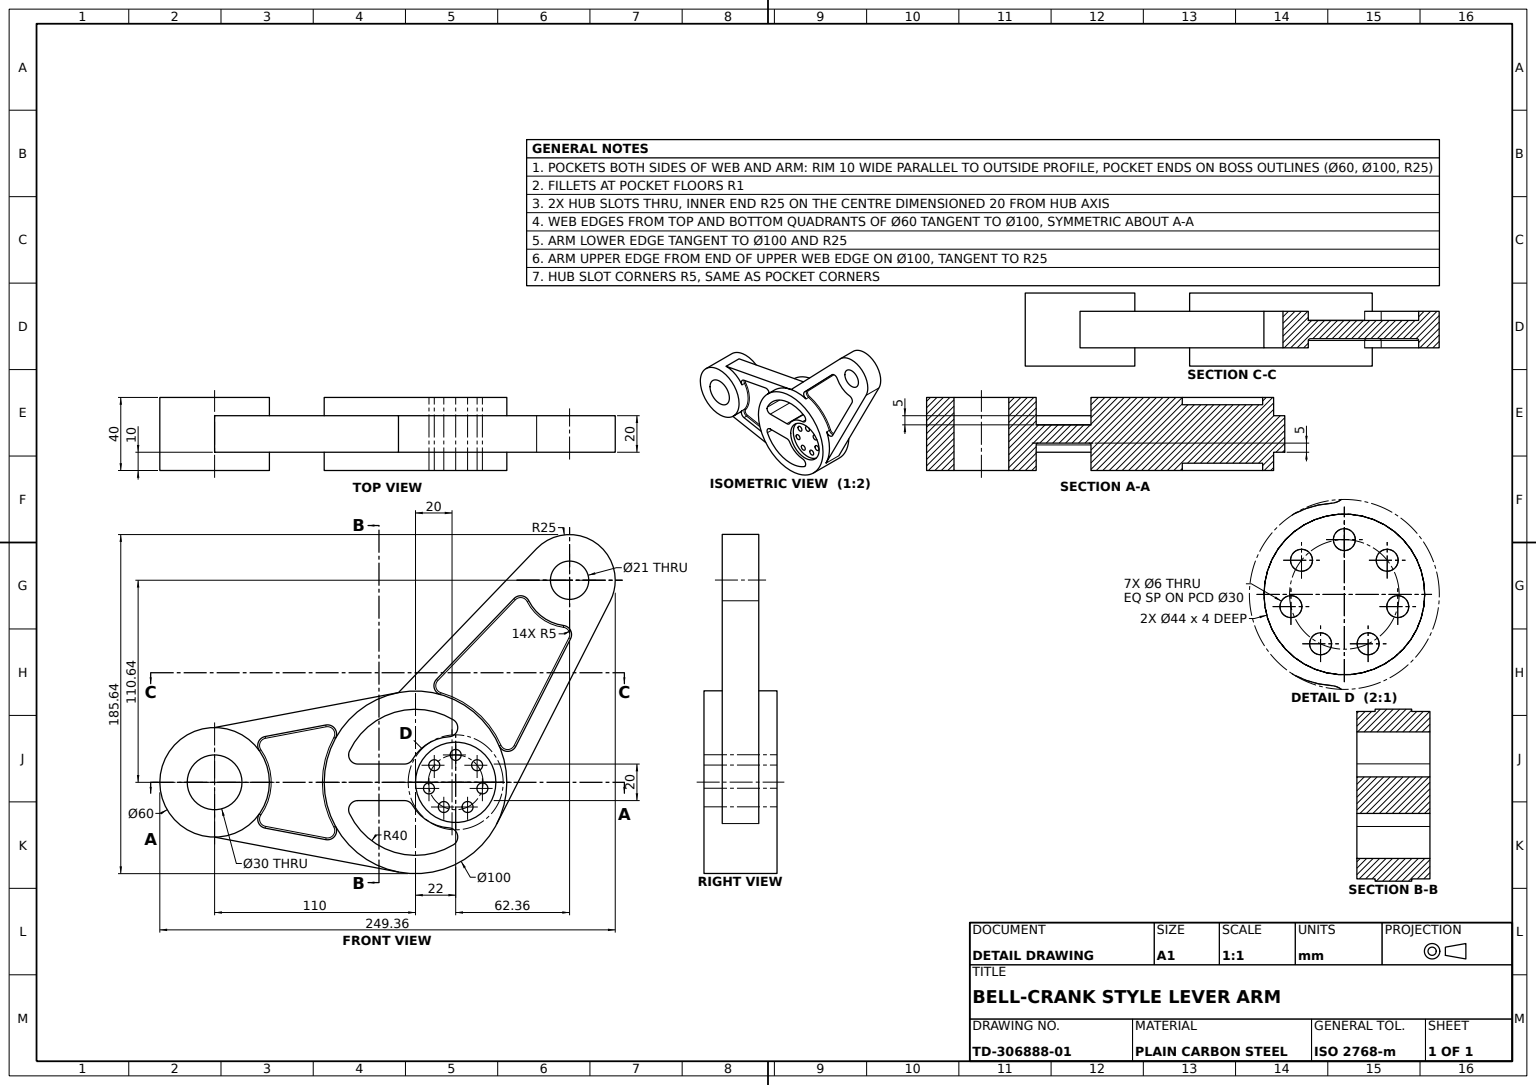
solid
v1 (18.491743913,-13.514533019,4)
v2 (18.491743913,-13.514533019,36)
e1 v1 v2 LINE
v3 (12.491743913,-13.514533019,36)
e2 v2 v3 CIRCLE(AX(P(15.491743913,-13.514533019,36),D(0,0,1),D(1,0,0)),3)
v4 (12.491743913,-13.514533019,4)
e3 v4 v3 LINE
e4 v4 v1 CIRCLE(AX(P(15.491743913,-13.514533019,4),D(0,0,-1),D(-1,0,0)),3)
face CYL(AX(P(15.491743913,-13.514533019,-4),D(0,0,1),D(1,0,0)),3) rev [e1 e2 -e3 e4]
v5 (54.673235414,99.92377456,25)
v6 (12.193310999,55.662253979,25)
e5 v5 v6 LINE
v7 (53.95175742,100.616211925,26)
e6 v7 v5 CIRCLE(AX(P(54.673235414,99.92377456,26),D(-0.692437365,-0.721477994,0),D(0.721477994,-0.692437365,0)),1)
v8 (11.471833004,56.354691343,26)
e7 v8 v7 LINE
e8 v8 v6 CIRCLE(AX(P(12.193310999,55.662253979,26),D(-0.692437365,-0.721477994,0),D(0.721477994,-0.692437365,0)),1)
face CYL(AX(P(12.193310999,55.662253979,26),D(-0.692437365,-0.721477994,0),D(0.721477994,-0.692437365,0)),1) rev [-e5 -e6 -e7 e8]
v9 (-36.622776602,15,40)
v10 (-36.622776602,15,0)
e9 v9 v10 LINE
v11 (-31.622776602,10,40)
e10 v11 v9 CIRCLE(AX(P(-31.622776602,15,40),D(0,0,-1),D(1,0,0)),5)
v12 (-31.622776602,10,0)
e11 v11 v12 LINE
e12 v12 v10 CIRCLE(AX(P(-31.622776602,15,0),D(0,0,-1),D(1,0,0)),5)
face CYL(AX(P(-31.622776602,15,40),D(0,0,-1),D(-1,0,0)),5) rev [-e9 -e10 e11 e12]
v13 (10.376081317,-3.337814009,36)
v14 (4.376081317,-3.337814009,36)
e13 v13 v14 CIRCLE(AX(P(7.376081317,-3.337814009,36),D(0,0,1),D(1,0,0)),3)
e14 v14 v13 CIRCLE(AX(P(7.376081317,-3.337814009,36),D(0,0,1),D(1,0,0)),3)
e15 v3 v2 CIRCLE(AX(P(15.491743913,-13.514533019,36),D(0,0,1),D(1,0,0)),3)
v15 (13.272527763,9.352347028,36)
v16 (7.272527763,9.352347028,36)
e16 v15 v16 CIRCLE(AX(P(10.272527763,9.352347028,36),D(0,0,1),D(1,0,0)),3)
e17 v16 v15 CIRCLE(AX(P(10.272527763,9.352347028,36),D(0,0,1),D(1,0,0)),3)
v17 (39.623918683,-3.337814009,36)
v18 (33.623918683,-3.337814009,36)
e18 v17 v18 CIRCLE(AX(P(36.623918683,-3.337814009,36),D(0,0,1),D(1,0,0)),3)
e19 v18 v17 CIRCLE(AX(P(36.623918683,-3.337814009,36),D(0,0,1),D(1,0,0)),3)
v19 (31.508256087,-13.514533019,36)
v20 (25.508256087,-13.514533019,36)
e20 v19 v20 CIRCLE(AX(P(28.508256087,-13.514533019,36),D(0,0,1),D(1,0,0)),3)
e21 v20 v19 CIRCLE(AX(P(28.508256087,-13.514533019,36),D(0,0,1),D(1,0,0)),3)
v21 (25,15,36)
v22 (19,15,36)
e22 v21 v22 CIRCLE(AX(P(22,15,36),D(0,0,1),D(1,0,0)),3)
e23 v22 v21 CIRCLE(AX(P(22,15,36),D(0,0,1),D(1,0,0)),3)
v23 (0,0,36)
v24 (44,0,36)
e24 v23 v24 CIRCLE(AX(P(22,0,36),D(0,0,1),D(1,0,0)),22)
e25 v24 v23 CIRCLE(AX(P(22,0,36),D(0,0,1),D(1,0,0)),22)
v25 (36.727472237,9.352347028,36)
v26 (30.727472237,9.352347028,36)
e26 v25 v26 CIRCLE(AX(P(33.727472237,9.352347028,36),D(0,0,1),D(1,0,0)),3)
e27 v26 v25 CIRCLE(AX(P(33.727472237,9.352347028,36),D(0,0,1),D(1,0,0)),3)
face PLANE(AX(P(22,0,36),D(0,0,1),D(1,0,0))) [-e13 -e14] [-e2 -e15] [-e16 -e17] [-e18 -e19] [-e20 -e21] [-e22 -e23] [e24 e25] [-e26 -e27]
v27 (81.094875761,85.850138645,30)
v28 (84.898130502,78.625049023,30)
e28 v27 v28 CIRCLE(AX(P(80.442048198,80.892940225,30),D(0,0,-1),D(1,0,0)),5)
v29 (81.094875761,85.850138645,26)
e29 v27 v29 LINE
v30 (85.442048198,80.892940225,26)
e30 v29 v30 CIRCLE(AX(P(80.442048198,80.892940225,26),D(0,0,-1),D(1,0,0)),5)
v31 (84.898130502,78.625049023,26)
e31 v30 v31 CIRCLE(AX(P(80.442048198,80.892940225,26),D(0,0,-1),D(1,0,0)),5)
e32 v28 v31 LINE
face CYL(AX(P(80.442048198,80.892940225,30),D(0,0,-1),D(-1,0,0)),5) rev [-e28 e29 e30 e31 -e32]
v32 (53.95175742,100.616211925,30)
e33 v32 v7 LINE
v33 (62.025791755,99.401042709,26)
e34 v7 v33 CIRCLE(AX(P(57.559147391,97.154025102,26),D(0,0,-1),D(1,0,0)),5)
v34 (62.025791755,99.401042709,30)
e35 v34 v33 LINE
e36 v32 v34 CIRCLE(AX(P(57.559147391,97.154025102,30),D(0,0,-1),D(1,0,0)),5)
face CYL(AX(P(57.559147391,97.154025102,30),D(0,0,-1),D(-1,0,0)),5) rev [e33 e34 -e35 -e36]
v35 (-82.326208539,25.077710319,30)
v36 (-82.326208539,25.077710319,26)
e37 v35 v36 LINE
v37 (-49.145510288,31.38022974,26)
e38 v36 v37 LINE
v38 (-49.145510288,31.38022974,30)
e39 v38 v37 LINE
e40 v35 v38 LINE
face PLANE(AX(P(-7.464353139,39.297371823,30),D(-0.186608828,0.982434296,0),D(-0.982434296,-0.186608828,0))) rev [e37 e38 -e39 -e40]
v39 (44,0,4)
v40 (44,0,0)
e41 v39 v40 LINE
v41 (0,0,4)
e42 v41 v39 CIRCLE(AX(P(22,0,4),D(0,0,-1),D(-1,0,0)),22)
v42 (0,0,0)
e43 v41 v42 LINE
e44 v42 v40 CIRCLE(AX(P(22,0,0),D(0,0,-1),D(-1,0,0)),22)
face CYL(AX(P(22,0,4),D(0,0,-1),D(-1,0,0)),22) rev [-e41 -e42 e43 e44]
v43 (-82.326208539,-25.077710319,26)
v44 (-86.393164396,-20.165538841,26)
e45 v43 v44 CIRCLE(AX(P(-81.393164396,-20.165538841,26),D(0,0,-1),D(-1,0,0)),5)
v45 (-86.393164396,-20.165538841,30)
e46 v45 v44 LINE
v46 (-82.326208539,-25.077710319,30)
e47 v46 v45 CIRCLE(AX(P(-81.393164396,-20.165538841,30),D(0,0,-1),D(1,0,0)),5)
e48 v46 v43 LINE
face CYL(AX(P(-81.393164396,-20.165538841,30),D(0,0,-1),D(-1,0,0)),5) rev [e45 -e46 -e47 e48]
v47 (-49.145510288,-31.38022974,30)
e49 v46 v47 LINE
v48 (-85.479855197,-17.284747578,30)
e50 v45 v48 CIRCLE(AX(P(-81.393164396,-20.165538841,30),D(0,0,-1),D(1,0,0)),5)
v49 (-110,-30,30)
e51 v48 v49 CIRCLE(AX(P(-110,0,30),D(0,0,-1),D(1,0,0)),30)
v50 (-9.330441424,-49.121714779,30)
e52 v49 v50 LINE
v51 (-43.829514678,-24.061871148,30)
e53 v51 v50 CIRCLE(AX(P(0,0,30),D(0,0,1),D(1,0,0)),50)
e54 v47 v51 CIRCLE(AX(P(-48.212466145,-26.468058263,30),D(0,0,1),D(1,0,0)),5)
face PLANE(AX(P(0,0,30),D(0,0,1),D(1,0,0))) [-e49 e47 e50 e51 e52 -e53 -e54]
v52 (-86.393164396,20.165538841,26)
e55 v52 v36 CIRCLE(AX(P(-81.393164396,20.165538841,26),D(0,0,-1),D(-1,0,0)),5)
v53 (-86.393164396,20.165538841,30)
e56 v35 v53 CIRCLE(AX(P(-81.393164396,20.165538841,30),D(0,0,1),D(1,0,0)),5)
e57 v53 v52 LINE
face CYL(AX(P(-81.393164396,20.165538841,30),D(0,0,-1),D(-1,0,0)),5) rev [e55 -e37 e56 e57]
v54 (33.623918683,-3.337814009,4)
e58 v54 v18 LINE
v55 (39.623918683,-3.337814009,4)
e59 v54 v55 CIRCLE(AX(P(36.623918683,-3.337814009,4),D(0,0,-1),D(-1,0,0)),3)
e60 v55 v17 LINE
face CYL(AX(P(36.623918683,-3.337814009,-4),D(0,0,1),D(1,0,0)),3) rev [e18 -e58 e59 e60]
v56 (-85.479855197,-17.284747578,15)
v57 (-85.479855197,-17.284747578,10)
e61 v56 v57 LINE
v58 (-86.393164396,-20.165538841,15)
e62 v56 v58 CIRCLE(AX(P(-81.393164396,-20.165538841,15),D(0,0,1),D(1,0,0)),5)
v59 (-86.393164396,-20.165538841,10)
e63 v58 v59 LINE
e64 v59 v57 CIRCLE(AX(P(-81.393164396,-20.165538841,10),D(0,0,-1),D(1,0,0)),5)
face CYL(AX(P(-81.393164396,-20.165538841,30),D(0,0,-1),D(-1,0,0)),5) rev [-e61 e62 e63 e64]
v60 (11.471833004,56.354691343,30)
v61 (10.079222976,52.892504521,30)
e65 v60 v61 CIRCLE(AX(P(15.079222976,52.892504521,30),D(0,0,1),D(1,0,0)),5)
v62 (10.079222976,52.892504521,26)
e66 v61 v62 LINE
e67 v62 v8 CIRCLE(AX(P(15.079222976,52.892504521,26),D(0,0,-1),D(1,0,0)),5)
e68 v60 v8 LINE
face CYL(AX(P(15.079222976,52.892504521,30),D(0,0,-1),D(-1,0,0)),5) rev [e65 e66 e67 -e68]
v63 (11.471833004,56.354691343,15)
v64 (11.471833004,56.354691343,10)
e69 v63 v64 LINE
v65 (10.079222976,52.892504521,15)
e70 v63 v65 CIRCLE(AX(P(15.079222976,52.892504521,15),D(0,0,1),D(1,0,0)),5)
v66 (10.079222976,52.892504521,10)
e71 v65 v66 LINE
e72 v64 v66 CIRCLE(AX(P(15.079222976,52.892504521,10),D(0,0,1),D(1,0,0)),5)
face CYL(AX(P(15.079222976,52.892504521,30),D(0,0,-1),D(-1,0,0)),5) rev [-e69 e70 e71 -e72]
v67 (-85.393164396,-20.165538841,25)
v68 (-82.13959971,-24.095276023,25)
e73 v67 v68 CIRCLE(AX(P(-81.393164396,-20.165538841,25),D(0,0,1),D(-1,0,0)),4)
e74 v44 v67 CIRCLE(AX(P(-85.393164396,-20.165538841,26),D(0,-1,0),D(0,0,-1)),1)
e75 v68 v43 CIRCLE(AX(P(-82.13959971,-24.095276023,26),D(-0.982434296,0.186608828,0),D(-0.186608828,-0.982434296,0)),1)
face TORUS(AX(P(-81.393164396,-20.165538841,26),D(0,0,-1),D(-1,0,0)),4,1) rev [-e73 -e74 -e45 -e75]
v69 (-36.140316116,-17.142857143,40)
v70 (-36.140316116,-17.142857143,0)
e76 v69 v70 LINE
v71 (-36.622776602,-15,0)
e77 v71 v70 CIRCLE(AX(P(-31.622776602,-15,0),D(0,0,1),D(1,0,0)),5)
v72 (-36.622776602,-15,40)
e78 v72 v71 LINE
e79 v72 v69 CIRCLE(AX(P(-31.622776602,-15,40),D(0,0,1),D(1,0,0)),5)
face CYL(AX(P(-31.622776602,-15,40),D(0,0,-1),D(-1,0,0)),5) rev [e76 -e77 -e78 e79]
v73 (-36.140316116,17.142857143,40)
v74 (-36.140316116,17.142857143,0)
e80 v73 v74 LINE
v75 (20.714285714,34.218684477,0)
e81 v75 v74 CIRCLE(AX(P(0,0,0),D(0,0,1),D(1,0,0)),40)
v76 (20.714285714,34.218684477,40)
e82 v76 v75 LINE
e83 v76 v73 CIRCLE(AX(P(0,0,40),D(0,0,1),D(1,0,0)),40)
face CYL(AX(P(0,0,40),D(0,0,-1),D(-1,0,0)),40) rev [e80 -e81 -e82 e83]
v77 (13.272527763,9.352347028,4)
e84 v77 v15 LINE
v78 (7.272527763,9.352347028,4)
e85 v77 v78 CIRCLE(AX(P(10.272527763,9.352347028,4),D(0,0,-1),D(-1,0,0)),3)
e86 v78 v16 LINE
face CYL(AX(P(10.272527763,9.352347028,-4),D(0,0,1),D(1,0,0)),3) rev [e17 -e84 e85 e86]
v79 (-85.479855197,17.284747578,30)
e87 v53 v79 CIRCLE(AX(P(-81.393164396,20.165538841,30),D(0,0,1),D(1,0,0)),5)
v80 (-85.479855197,17.284747578,26)
e88 v79 v80 LINE
e89 v80 v52 CIRCLE(AX(P(-81.393164396,20.165538841,26),D(0,0,-1),D(-1,0,0)),5)
face CYL(AX(P(-81.393164396,20.165538841,30),D(0,0,-1),D(-1,0,0)),5) rev [e87 e88 e89 -e57]
v81 (-82.326208539,-25.077710319,15)
v82 (-49.145510288,-31.38022974,15)
e90 v81 v82 LINE
v83 (-49.145510288,-31.38022974,10)
e91 v82 v83 LINE
v84 (-82.326208539,-25.077710319,10)
e92 v84 v83 LINE
e93 v81 v84 LINE
face PLANE(AX(P(-7.464353139,-39.297371823,30),D(0.186608828,0.982434296,0),D(-0.982434296,0.186608828,0))) [e90 e91 -e92 -e93]
v85 (13.708384523,48.084095019,30)
e94 v61 v85 CIRCLE(AX(P(15.079222976,52.892504521,30),D(0,0,1),D(1,0,0)),5)
v86 (13.708384523,48.084095019,26)
e95 v85 v86 LINE
e96 v86 v62 CIRCLE(AX(P(15.079222976,52.892504521,26),D(0,0,-1),D(1,0,0)),5)
face CYL(AX(P(15.079222976,52.892504521,30),D(0,0,-1),D(-1,0,0)),5) rev [-e66 e94 e95 e96]
e97 v78 v77 CIRCLE(AX(P(10.272527763,9.352347028,4),D(0,0,-1),D(-1,0,0)),3)
face CYL(AX(P(10.272527763,9.352347028,-4),D(0,0,1),D(1,0,0)),3) rev [-e86 e97 e84 e16]
v87 (-5.980762114,-10,40)
v88 (-5.980762114,-10,0)
e98 v87 v88 LINE
v89 (-31.622776602,-10,40)
e99 v87 v89 LINE
v90 (-31.622776602,-10,0)
e100 v89 v90 LINE
e101 v88 v90 LINE
face PLANE(AX(P(0,-10,40),D(0,-1,0),D(1,0,0))) [-e98 e99 e100 -e101]
v91 (13.708384523,48.084095019,15)
v92 (13.708384523,48.084095019,10)
e102 v91 v92 LINE
e103 v66 v92 CIRCLE(AX(P(15.079222976,52.892504521,10),D(0,0,1),D(1,0,0)),5)
e104 v65 v91 CIRCLE(AX(P(15.079222976,52.892504521,15),D(0,0,1),D(1,0,0)),5)
face CYL(AX(P(15.079222976,52.892504521,30),D(0,0,-1),D(-1,0,0)),5) rev [e102 -e103 -e71 e104]
v93 (45.851155545,19.941703417,26)
v94 (46.768178656,20.340537485,25)
e105 v93 v94 CIRCLE(AX(P(46.768178656,20.340537485,26),D(0.398834068,-0.917023111,0),D(0.917023111,0.398834068,0)),1)
v95 (54.892353403,19.667982557,26)
e106 v95 v93 CIRCLE(AX(P(50.4362711,21.935873759,26),D(0,0,-1),D(1,0,0)),5)
v96 (54.001136943,20.121560797,25)
e107 v96 v95 CIRCLE(AX(P(54.001136943,20.121560797,26),D(-0.45357824,-0.891216461,0),D(0.891216461,-0.45357824,0)),1)
e108 v94 v96 CIRCLE(AX(P(50.4362711,21.935873759,25),D(0,0,1),D(1,0,0)),4)
face TORUS(AX(P(50.4362711,21.935873759,26),D(0,0,1),D(1,0,0)),4,1) rev [-e105 -e106 -e107 -e108]
v97 (-50,0,26)
v98 (-43.829514678,-24.061871148,26)
e109 v97 v98 CIRCLE(AX(P(0,0,26),D(0,0,1),D(-1,0,0)),50)
v99 (-51,0,25)
e110 v99 v97 CIRCLE(AX(P(-51,0,26),D(0,-1,0),D(0,0,-1)),1)
v100 (-44.706104971,-24.543108571,25)
e111 v100 v99 CIRCLE(AX(P(0,0,25),D(0,0,-1),D(-1,0,0)),51)
e112 v100 v98 CIRCLE(AX(P(-44.706104971,-24.543108571,26),D(0.481237423,-0.876590294,0),D(0.876590294,0.481237423,0)),1)
face TORUS(AX(P(0,0,26),D(0,0,-1),D(-1,0,0)),51,1) rev [-e109 -e110 -e111 e112]
v101 (-80,0,15)
e113 v101 v56 CIRCLE(AX(P(-110,0,15),D(0,0,-1),D(-1,0,0)),30)
v102 (-85.479855197,17.284747578,15)
e114 v102 v101 CIRCLE(AX(P(-110,0,15),D(0,0,-1),D(-1,0,0)),30)
v103 (-86.393164396,20.165538841,15)
e115 v103 v102 CIRCLE(AX(P(-81.393164396,20.165538841,15),D(0,0,1),D(-1,0,0)),5)
v104 (-82.326208539,25.077710319,15)
e116 v104 v103 CIRCLE(AX(P(-81.393164396,20.165538841,15),D(0,0,1),D(-1,0,0)),5)
v105 (-49.145510288,31.38022974,15)
e117 v105 v104 LINE
v106 (-43.829514678,24.061871148,15)
e118 v106 v105 CIRCLE(AX(P(-48.212466145,26.468058263,15),D(0,0,1),D(-1,0,0)),5)
v107 (-50,0,15)
e119 v107 v106 CIRCLE(AX(P(0,0,15),D(0,0,-1),D(1,0,0)),50)
v108 (-43.829514678,-24.061871148,15)
e120 v108 v107 CIRCLE(AX(P(0,0,15),D(0,0,-1),D(1,0,0)),50)
e121 v82 v108 CIRCLE(AX(P(-48.212466145,-26.468058263,15),D(0,0,1),D(1,0,0)),5)
e122 v58 v81 CIRCLE(AX(P(-81.393164396,-20.165538841,15),D(0,0,1),D(1,0,0)),5)
face PLANE(AX(P(-110,0,15),D(0,0,-1),D(-1,0,0))) [-e113 -e114 -e115 -e116 -e117 -e118 -e119 -e120 -e121 -e90 -e122 -e62]
v109 (-80,0,0)
v110 (-140,0,0)
e123 v109 v110 CIRCLE(AX(P(-110,0,0),D(0,0,1),D(1,0,0)),30)
e124 v110 v109 CIRCLE(AX(P(-110,0,0),D(0,0,1),D(1,0,0)),30)
v111 (-95,0,0)
v112 (-125,0,0)
e125 v111 v112 CIRCLE(AX(P(-110,0,0),D(0,0,1),D(1,0,0)),15)
e126 v112 v111 CIRCLE(AX(P(-110,0,0),D(0,0,1),D(1,0,0)),15)
face PLANE(AX(P(-110,0,0),D(0,0,1),D(1,0,0))) rev [-e123 -e124] [e125 e126]
v113 (-86.393164396,20.165538841,10)
e127 v103 v113 LINE
v114 (-82.326208539,25.077710319,10)
e128 v114 v113 CIRCLE(AX(P(-81.393164396,20.165538841,10),D(0,0,1),D(1,0,0)),5)
e129 v104 v114 LINE
face CYL(AX(P(-81.393164396,20.165538841,30),D(0,0,-1),D(-1,0,0)),5) rev [e116 e127 -e128 -e129]
e130 v1 v4 CIRCLE(AX(P(15.491743913,-13.514533019,4),D(0,0,-1),D(-1,0,0)),3)
face CYL(AX(P(15.491743913,-13.514533019,-4),D(0,0,1),D(1,0,0)),3) rev [-e1 e130 e3 e15]
v115 (-80,0,40)
v116 (-140,0,40)
e131 v115 v116 CIRCLE(AX(P(-110,0,40),D(0,0,1),D(1,0,0)),30)
e132 v116 v115 CIRCLE(AX(P(-110,0,40),D(0,0,1),D(1,0,0)),30)
v117 (-95,0,40)
v118 (-125,0,40)
e133 v117 v118 CIRCLE(AX(P(-110,0,40),D(0,0,1),D(1,0,0)),15)
e134 v118 v117 CIRCLE(AX(P(-110,0,40),D(0,0,1),D(1,0,0)),15)
face PLANE(AX(P(-110,0,40),D(0,0,1),D(1,0,0))) [e131 e132] [-e133 -e134]
v119 (61.132462882,98.951639187,25)
e135 v119 v33 CIRCLE(AX(P(61.132462882,98.951639187,26),D(0.449403521,-0.893328873,0),D(0.893328873,0.449403521,0)),1)
e136 v119 v5 CIRCLE(AX(P(57.559147391,97.154025102,25),D(0,0,1),D(1,0,0)),4)
face TORUS(AX(P(57.559147391,97.154025102,26),D(0,0,1),D(1,0,0)),4,1) rev [e135 -e34 e6 -e136]
v120 (4.376081317,-3.337814009,4)
e137 v120 v14 LINE
v121 (10.376081317,-3.337814009,4)
e138 v121 v13 LINE
e139 v121 v120 CIRCLE(AX(P(7.376081317,-3.337814009,4),D(0,0,-1),D(-1,0,0)),3)
face CYL(AX(P(7.376081317,-3.337814009,-4),D(0,0,1),D(1,0,0)),3) rev [e137 e14 -e138 e139]
v122 (-9.330441424,49.121714779,30)
v123 (-9.330441424,49.121714779,10)
e140 v122 v123 LINE
v124 (-110,30,10)
e141 v124 v123 LINE
v125 (-110,30,30)
e142 v125 v124 LINE
e143 v125 v122 LINE
face PLANE(AX(P(-9.330441424,49.121714779,30),D(-0.186608828,0.982434296,0),D(-0.982434296,-0.186608828,0))) [e140 -e141 -e142 e143]
v126 (-43.829514678,-24.061871148,10)
e144 v83 v126 CIRCLE(AX(P(-48.212466145,-26.468058263,10),D(0,0,1),D(1,0,0)),5)
v127 (-9.330441424,-49.121714779,10)
e145 v126 v127 CIRCLE(AX(P(0,0,10),D(0,0,1),D(1,0,0)),50)
v128 (-110,-30,10)
e146 v128 v127 LINE
e147 v57 v128 CIRCLE(AX(P(-110,0,10),D(0,0,-1),D(1,0,0)),30)
e148 v84 v59 CIRCLE(AX(P(-81.393164396,-20.165538841,10),D(0,0,-1),D(1,0,0)),5)
face PLANE(AX(P(0,0,10),D(0,0,1),D(1,0,0))) rev [e92 e144 e145 -e146 -e147 -e64 -e148]
v129 (53.95175742,100.616211925,10)
v130 (62.025791755,99.401042709,10)
e149 v129 v130 CIRCLE(AX(P(57.559147391,97.154025102,10),D(0,0,-1),D(1,0,0)),5)
e150 v64 v129 LINE
e151 v92 v123 CIRCLE(AX(P(0,0,10),D(0,0,1),D(1,0,0)),50)
v131 (66.322063718,127.947064858,10)
e152 v123 v131 LINE
v132 (109.359013574,110.636130744,10)
e153 v131 v132 CIRCLE(AX(P(84.359013574,110.636130744,10),D(0,0,-1),D(-1,0,0)),25)
v133 (106.639425092,99.296674734,10)
e154 v132 v133 CIRCLE(AX(P(84.359013574,110.636130744,10),D(0,0,-1),D(-1,0,0)),25)
v134 (44.560823036,-22.67891202,10)
e155 v133 v134 LINE
v135 (50,0,10)
e156 v134 v135 CIRCLE(AX(P(0,0,10),D(0,0,1),D(1,0,0)),50)
v136 (45.851155545,19.941703417,10)
e157 v135 v136 CIRCLE(AX(P(0,0,10),D(0,0,1),D(1,0,0)),50)
v137 (54.892353403,19.667982557,10)
e158 v136 v137 CIRCLE(AX(P(50.4362711,21.935873759,10),D(0,0,1),D(1,0,0)),5)
v138 (84.898130502,78.625049023,10)
e159 v138 v137 LINE
v139 (81.094875761,85.850138645,10)
e160 v139 v138 CIRCLE(AX(P(80.442048198,80.892940225,10),D(0,0,-1),D(1,0,0)),5)
e161 v139 v130 CIRCLE(AX(P(84.359013574,110.636130744,10),D(0,0,-1),D(-1,0,0)),25)
v140 (73.859013574,110.636130744,10)
v141 (94.859013574,110.636130744,10)
e162 v140 v141 CIRCLE(AX(P(84.359013574,110.636130744,10),D(0,0,-1),D(-1,0,0)),10.5)
e163 v141 v140 CIRCLE(AX(P(84.359013574,110.636130744,10),D(0,0,-1),D(-1,0,0)),10.5)
face PLANE(AX(P(0,0,10),D(0,0,1),D(1,0,0))) rev [-e149 -e150 e72 e103 e151 e152 e153 e154 e155 e156 e157 e158 -e159 -e160 e161] [-e162 -e163]
e164 v60 v32 LINE
face PLANE(AX(P(-22.182143151,21.289276827,30),D(-0.721477994,0.692437365,0),D(-0.692437365,-0.721477994,0))) rev [e68 e7 -e33 -e164]
v142 (13.982552214,49.045776919,25)
e165 v142 v94 CIRCLE(AX(P(0,0,25),D(0,0,-1),D(1,0,0)),51)
e166 v86 v142 CIRCLE(AX(P(13.982552214,49.045776919,26),D(0.9616819,-0.27416769,0),D(0.27416769,0.9616819,0)),1)
e167 v93 v86 CIRCLE(AX(P(0,0,26),D(0,0,1),D(1,0,0)),50)
face TORUS(AX(P(0,0,26),D(0,0,1),D(1,0,0)),51,1) rev [e105 -e165 -e166 -e167]
e168 v40 v42 CIRCLE(AX(P(22,0,0),D(0,0,-1),D(-1,0,0)),22)
e169 v39 v41 CIRCLE(AX(P(22,0,4),D(0,0,-1),D(-1,0,0)),22)
face CYL(AX(P(22,0,4),D(0,0,-1),D(-1,0,0)),22) rev [e168 -e43 -e169 e41]
v143 (45.851155545,19.941703417,15)
e170 v91 v143 CIRCLE(AX(P(0,0,15),D(0,0,-1),D(-1,0,0)),50)
e171 v143 v136 LINE
v144 (50,0,0)
e172 v135 v144 LINE
v145 (-50,0,0)
e173 v144 v145 CIRCLE(AX(P(0,0,0),D(0,0,1),D(1,0,0)),50)
e174 v107 v145 LINE
v146 (-43.829514678,24.061871148,10)
e175 v106 v146 LINE
e176 v123 v146 CIRCLE(AX(P(0,0,10),D(0,0,1),D(1,0,0)),50)
face CYL(AX(P(0,0,40),D(0,0,-1),D(-1,0,0)),50) [-e151 -e102 e170 e171 -e157 e172 e173 -e174 e119 e175 -e176]
v147 (-85.479855197,17.284747578,10)
e177 v113 v147 CIRCLE(AX(P(-81.393164396,20.165538841,10),D(0,0,1),D(1,0,0)),5)
e178 v124 v147 CIRCLE(AX(P(-110,0,10),D(0,0,-1),D(1,0,0)),30)
v148 (-49.145510288,31.38022974,10)
e179 v148 v146 CIRCLE(AX(P(-48.212466145,26.468058263,10),D(0,0,-1),D(1,0,0)),5)
e180 v114 v148 LINE
face PLANE(AX(P(0,0,10),D(0,0,1),D(1,0,0))) rev [e177 -e178 e141 e176 -e179 -e180 e128]
v149 (94.859013574,110.636130744,30)
e181 v141 v149 LINE
v150 (73.859013574,110.636130744,30)
e182 v149 v150 CIRCLE(AX(P(84.359013574,110.636130744,30),D(0,0,1),D(1,0,0)),10.5)
e183 v140 v150 LINE
face CYL(AX(P(84.359013574,110.636130744,0),D(0,0,1),D(1,0,0)),10.5) rev [e181 e182 -e183 e162]
v151 (54.892353403,19.667982557,30)
e184 v151 v95 LINE
v152 (45.851155545,19.941703417,30)
e185 v152 v93 LINE
e186 v152 v151 CIRCLE(AX(P(50.4362711,21.935873759,30),D(0,0,1),D(1,0,0)),5)
face CYL(AX(P(50.4362711,21.935873759,30),D(0,0,-1),D(-1,0,0)),5) rev [e184 e106 -e185 e186]
v153 (-85.393164396,20.165538841,25)
v154 (-84.662517037,17.86090583,25)
e187 v153 v154 CIRCLE(AX(P(-81.393164396,20.165538841,25),D(0,0,1),D(-1,0,0)),4)
e188 v52 v153 CIRCLE(AX(P(-85.393164396,20.165538841,26),D(0,-1,0),D(0,0,-1)),1)
e189 v80 v154 CIRCLE(AX(P(-84.662517037,17.86090583,26),D(0.576158253,-0.81733816,0),D(0.81733816,0.576158253,0)),1)
face TORUS(AX(P(-81.393164396,20.165538841,26),D(0,0,-1),D(-1,0,0)),4,1) rev [-e187 -e188 -e89 e189]
v155 (-85.479855197,-17.284747578,26)
e190 v44 v155 CIRCLE(AX(P(-81.393164396,-20.165538841,26),D(0,0,-1),D(-1,0,0)),5)
e191 v48 v155 LINE
face CYL(AX(P(-81.393164396,-20.165538841,30),D(0,0,-1),D(-1,0,0)),5) rev [e46 e190 -e191 -e50]
v156 (-82.13959971,24.095276023,25)
e192 v36 v156 CIRCLE(AX(P(-82.13959971,24.095276023,26),D(-0.982434296,-0.186608828,0),D(0.186608828,-0.982434296,0)),1)
v157 (-48.958901459,30.397795445,25)
e193 v157 v156 LINE
e194 v37 v157 CIRCLE(AX(P(-48.958901459,30.397795445,26),D(-0.982434296,-0.186608828,0),D(0.186608828,-0.982434296,0)),1)
face CYL(AX(P(-113.447230275,18.148537103,26),D(0.982434296,0.186608828,0),D(-0.186608828,0.982434296,0)),1) rev [-e38 e192 -e193 -e194]
e195 v120 v121 CIRCLE(AX(P(7.376081317,-3.337814009,4),D(0,0,-1),D(-1,0,0)),3)
face CYL(AX(P(7.376081317,-3.337814009,-4),D(0,0,1),D(1,0,0)),3) rev [e138 e13 -e137 e195]
e196 v102 v147 LINE
e197 v109 v101 LINE
e198 v110 v116 LINE
v158 (-80,0,26)
e199 v158 v115 LINE
e200 v158 v80 CIRCLE(AX(P(-110,0,26),D(0,0,1),D(-1,0,0)),30)
e201 v125 v79 CIRCLE(AX(P(-110,0,30),D(0,0,-1),D(1,0,0)),30)
face CYL(AX(P(-110,0,0),D(0,0,1),D(1,0,0)),30) [e178 -e196 e114 -e197 e123 e198 -e131 -e199 e200 -e88 -e201 e142]
v159 (84.442048198,80.892940225,25)
e202 v159 v30 CIRCLE(AX(P(84.442048198,80.892940225,26),D(0,-1,0),D(0,0,-1)),1)
v160 (84.006914041,79.078627264,25)
e203 v160 v159 CIRCLE(AX(P(80.442048198,80.892940225,25),D(0,0,1),D(1,0,0)),4)
e204 v160 v31 CIRCLE(AX(P(84.006914041,79.078627264,26),D(-0.45357824,-0.891216461,0),D(0.891216461,-0.45357824,0)),1)
face TORUS(AX(P(80.442048198,80.892940225,26),D(0,0,1),D(1,0,0)),4,1) rev [-e31 -e202 -e203 e204]
v161 (106.639425092,99.296674734,30)
e205 v161 v133 LINE
v162 (44.560823036,-22.67891202,30)
e206 v161 v162 LINE
e207 v162 v134 LINE
face PLANE(AX(P(44.560823036,-22.67891202,30),D(0.891216461,-0.45357824,0),D(0.45357824,0.891216461,0))) [-e155 -e205 e206 e207]
v163 (18.4375,-24.951124098,40)
v164 (18.4375,-24.951124098,0)
e208 v163 v164 LINE
v165 (20.714285714,-34.218684477,0)
e209 v164 v165 CIRCLE(AX(P(18.125,-29.941348918,0),D(0,0,-1),D(1,0,0)),5)
v166 (20.714285714,-34.218684477,40)
e210 v166 v165 LINE
e211 v163 v166 CIRCLE(AX(P(18.125,-29.941348918,40),D(0,0,-1),D(1,0,0)),5)
face CYL(AX(P(18.125,-29.941348918,40),D(0,0,-1),D(-1,0,0)),5) rev [e208 e209 -e210 -e211]
e212 v108 v126 LINE
face CYL(AX(P(-48.212466145,-26.468058263,30),D(0,0,-1),D(-1,0,0)),5) rev [-e91 e121 e212 -e144]
v167 (-1.650635095,-12.5,40)
e213 v163 v167 CIRCLE(AX(P(20,0,40),D(0,0,-1),D(1,0,0)),25)
v168 (-1.650635095,-12.5,0)
e214 v167 v168 LINE
e215 v164 v168 CIRCLE(AX(P(20,0,0),D(0,0,-1),D(1,0,0)),25)
face CYL(AX(P(20,0,40),D(0,0,-1),D(-1,0,0)),25) [-e208 e213 e214 -e215]
v169 (25,15,4)
v170 (19,15,4)
e216 v169 v170 CIRCLE(AX(P(22,15,4),D(0,0,-1),D(-1,0,0)),3)
e217 v170 v22 LINE
e218 v169 v21 LINE
face CYL(AX(P(22,15,-4),D(0,0,1),D(1,0,0)),3) rev [e216 e217 e23 -e218]
v171 (-43.829514678,24.061871148,30)
e219 v38 v171 CIRCLE(AX(P(-48.212466145,26.468058263,30),D(0,0,-1),D(1,0,0)),5)
e220 v122 v171 CIRCLE(AX(P(0,0,30),D(0,0,1),D(1,0,0)),50)
face PLANE(AX(P(0,0,30),D(0,0,1),D(1,0,0))) [e40 e219 -e220 -e143 e201 -e87 -e56]
e221 v6 v142 CIRCLE(AX(P(15.079222976,52.892504521,25),D(0,0,1),D(1,0,0)),4)
face TORUS(AX(P(15.079222976,52.892504521,26),D(0,0,1),D(1,0,0)),4,1) rev [-e67 -e96 e166 -e221 -e8]
v172 (54.892353403,19.667982557,15)
e222 v172 v137 LINE
v173 (84.898130502,78.625049023,15)
e223 v172 v173 LINE
e224 v173 v138 LINE
face PLANE(AX(P(35.648658428,-18.143129616,30),D(0.891216461,-0.45357824,0),D(0.45357824,0.891216461,0))) rev [e159 -e222 e223 e224]
e225 v28 v151 LINE
e226 v31 v95 LINE
face PLANE(AX(P(35.648658428,-18.143129616,30),D(0.891216461,-0.45357824,0),D(0.45357824,0.891216461,0))) rev [-e184 -e225 e32 e226]
e227 v156 v153 CIRCLE(AX(P(-81.393164396,20.165538841,25),D(0,0,1),D(-1,0,0)),4)
face TORUS(AX(P(-81.393164396,20.165538841,26),D(0,0,-1),D(-1,0,0)),4,1) rev [-e227 -e192 -e55 e188]
e228 v87 v167 CIRCLE(AX(P(-5.980762114,-15,40),D(0,0,-1),D(1,0,0)),5)
e229 v88 v168 CIRCLE(AX(P(-5.980762114,-15,0),D(0,0,-1),D(1,0,0)),5)
face CYL(AX(P(-5.980762114,-15,40),D(0,0,-1),D(-1,0,0)),5) rev [-e214 -e228 e98 e229]
e230 v51 v98 LINE
e231 v50 v127 LINE
e232 v145 v144 CIRCLE(AX(P(0,0,0),D(0,0,1),D(1,0,0)),50)
v174 (50,0,30)
e233 v162 v174 CIRCLE(AX(P(0,0,30),D(0,0,1),D(1,0,0)),50)
v175 (50,0,40)
e234 v175 v174 LINE
v176 (-50,0,40)
e235 v176 v175 CIRCLE(AX(P(0,0,40),D(0,0,1),D(1,0,0)),50)
e236 v176 v97 LINE
face CYL(AX(P(0,0,40),D(0,0,-1),D(-1,0,0)),50) [e109 -e230 e53 e231 -e145 -e212 e120 e174 e232 -e172 -e156 -e207 e233 -e234 -e235 e236]
e237 v150 v149 CIRCLE(AX(P(84.359013574,110.636130744,30),D(0,0,1),D(1,0,0)),10.5)
face CYL(AX(P(84.359013574,110.636130744,0),D(0,0,1),D(1,0,0)),10.5) rev [e237 -e181 e163 e183]
v177 (62.025791755,99.401042709,15)
e238 v177 v130 LINE
v178 (53.95175742,100.616211925,15)
e239 v177 v178 CIRCLE(AX(P(57.559147391,97.154025102,15),D(0,0,1),D(-1,0,0)),5)
e240 v178 v129 LINE
face CYL(AX(P(57.559147391,97.154025102,30),D(0,0,-1),D(-1,0,0)),5) rev [-e238 e239 e240 e149]
e241 v49 v128 LINE
e242 v155 v158 CIRCLE(AX(P(-110,0,26),D(0,0,1),D(-1,0,0)),30)
face CYL(AX(P(-110,0,0),D(0,0,1),D(1,0,0)),30) [e113 e61 e147 -e241 -e51 e191 e242 e199 -e132 -e198 e124 e197]
v179 (-44.706104971,24.543108571,25)
e243 v179 v157 CIRCLE(AX(P(-48.212466145,26.468058263,25),D(0,0,1),D(-1,0,0)),4)
v180 (-43.829514678,24.061871148,26)
e244 v179 v180 CIRCLE(AX(P(-44.706104971,24.543108571,26),D(-0.481237423,-0.876590294,0),D(0.876590294,-0.481237423,0)),1)
e245 v37 v180 CIRCLE(AX(P(-48.212466145,26.468058263,26),D(0,0,-1),D(-1,0,0)),5)
face TORUS(AX(P(-48.212466145,26.468058263,26),D(0,0,-1),D(-1,0,0)),4,1) rev [e194 -e243 e244 -e245]
e246 v96 v160 LINE
v181 (80.964310248,84.858698961,25)
e247 v159 v181 CIRCLE(AX(P(80.442048198,80.892940225,25),D(0,0,1),D(1,0,0)),4)
e248 v181 v119 CIRCLE(AX(P(84.359013574,110.636130744,25),D(0,0,-1),D(1,0,0)),26)
face PLANE(AX(P(15.079222976,52.892504521,25),D(0,0,1),D(1,0,0))) [e246 e203 e247 e248 e136 e5 e221 e165 e108]
v182 (-49.145510288,-31.38022974,26)
e249 v98 v182 CIRCLE(AX(P(-48.212466145,-26.468058263,26),D(0,0,-1),D(-1,0,0)),5)
e250 v47 v182 LINE
face CYL(AX(P(-48.212466145,-26.468058263,30),D(0,0,-1),D(-1,0,0)),5) rev [e54 e230 e249 -e250]
e251 v165 v70 CIRCLE(AX(P(0,0,0),D(0,0,-1),D(1,0,0)),40)
e252 v166 v69 CIRCLE(AX(P(0,0,40),D(0,0,-1),D(1,0,0)),40)
face CYL(AX(P(0,0,40),D(0,0,-1),D(-1,0,0)),40) rev [e251 -e76 -e252 e210]
v183 (31.508256087,-13.514533019,4)
v184 (25.508256087,-13.514533019,4)
e253 v183 v184 CIRCLE(AX(P(28.508256087,-13.514533019,4),D(0,0,-1),D(-1,0,0)),3)
e254 v184 v20 LINE
e255 v183 v19 LINE
face CYL(AX(P(28.508256087,-13.514533019,-4),D(0,0,1),D(1,0,0)),3) rev [e253 e254 e21 -e255]
v185 (109.359013574,110.636130744,30)
e256 v161 v185 CIRCLE(AX(P(84.359013574,110.636130744,30),D(0,0,1),D(1,0,0)),25)
e257 v132 v185 LINE
face CYL(AX(P(84.359013574,110.636130744,0),D(0,0,1),D(1,0,0)),25) [-e256 e205 -e154 e257]
e258 v178 v63 LINE
face PLANE(AX(P(-22.182143151,21.289276827,30),D(-0.721477994,0.692437365,0),D(-0.692437365,-0.721477994,0))) rev [-e240 e258 e69 e150]
e259 v181 v29 CIRCLE(AX(P(80.964310248,84.858698961,26),D(0.991439684,-0.130565513,0),D(0.130565513,0.991439684,0)),1)
face TORUS(AX(P(80.442048198,80.892940225,26),D(0,0,1),D(1,0,0)),4,1) rev [-e247 e202 -e30 -e259]
v186 (66.322063718,127.947064858,30)
e260 v185 v186 CIRCLE(AX(P(84.359013574,110.636130744,30),D(0,0,1),D(1,0,0)),25)
e261 v122 v186 LINE
e262 v85 v122 CIRCLE(AX(P(0,0,30),D(0,0,1),D(1,0,0)),50)
e263 v34 v27 CIRCLE(AX(P(84.359013574,110.636130744,30),D(0,0,1),D(1,0,0)),25)
e264 v174 v152 CIRCLE(AX(P(0,0,30),D(0,0,1),D(1,0,0)),50)
face PLANE(AX(P(0,0,30),D(0,0,1),D(1,0,0))) [e260 -e261 -e262 -e94 -e65 e164 e36 e263 e28 e225 -e186 -e264 -e233 -e206 e256] [-e182 -e237]
e265 v33 v29 CIRCLE(AX(P(84.359013574,110.636130744,26),D(0,0,1),D(1,0,0)),25)
face TORUS(AX(P(84.359013574,110.636130744,26),D(0,0,1),D(1,0,0)),26,1) rev [-e265 -e135 -e248 e259]
e266 v182 v43 LINE
v187 (-48.958901459,-30.397795445,25)
e267 v187 v182 CIRCLE(AX(P(-48.958901459,-30.397795445,26),D(-0.982434296,0.186608828,0),D(-0.186608828,-0.982434296,0)),1)
e268 v68 v187 LINE
face CYL(AX(P(-113.447230275,-18.148537103,26),D(0.982434296,-0.186608828,0),D(0.186608828,0.982434296,0)),1) rev [-e266 -e267 -e268 e75]
v188 (-84.662517037,-17.86090583,25)
e269 v188 v67 CIRCLE(AX(P(-81.393164396,-20.165538841,25),D(0,0,1),D(-1,0,0)),4)
e270 v155 v188 CIRCLE(AX(P(-84.662517037,-17.86090583,26),D(-0.576158253,-0.81733816,0),D(0.81733816,-0.576158253,0)),1)
face TORUS(AX(P(-81.393164396,-20.165538841,26),D(0,0,-1),D(-1,0,0)),4,1) rev [-e269 -e270 -e190 e74]
e271 v154 v188 CIRCLE(AX(P(-110,0,25),D(0,0,-1),D(-1,0,0)),31)
face TORUS(AX(P(-110,0,26),D(0,0,-1),D(-1,0,0)),31,1) rev [-e189 -e200 -e242 e270 -e271]
v189 (44,0,40)
e272 v24 v189 LINE
v190 (0,0,40)
e273 v23 v190 LINE
e274 v190 v189 CIRCLE(AX(P(22,0,40),D(0,0,1),D(1,0,0)),22)
face CYL(AX(P(22,0,36),D(0,0,1),D(1,0,0)),22) rev [-e272 -e24 e273 e274]
e275 v105 v148 LINE
face PLANE(AX(P(-7.464353139,39.297371823,30),D(-0.186608828,0.982434296,0),D(-0.982434296,-0.186608828,0))) rev [e129 e180 -e275 e117]
face PLANE(AX(P(-7.464353139,-39.297371823,30),D(0.186608828,0.982434296,0),D(-0.982434296,0.186608828,0))) [e250 e266 -e48 e49]
e276 v10 v74 CIRCLE(AX(P(-31.622776602,15,0),D(0,0,-1),D(1,0,0)),5)
e277 v9 v73 CIRCLE(AX(P(-31.622776602,15,40),D(0,0,-1),D(1,0,0)),5)
face CYL(AX(P(-31.622776602,15,40),D(0,0,-1),D(-1,0,0)),5) rev [e9 e276 -e80 -e277]
e278 v89 v72 CIRCLE(AX(P(-31.622776602,-15,40),D(0,0,1),D(1,0,0)),5)
e279 v90 v71 CIRCLE(AX(P(-31.622776602,-15,0),D(0,0,1),D(1,0,0)),5)
face CYL(AX(P(-31.622776602,-15,40),D(0,0,-1),D(-1,0,0)),5) rev [-e100 e278 e78 -e279]
face CYL(AX(P(-81.393164396,20.165538841,30),D(0,0,-1),D(-1,0,0)),5) rev [-e177 -e127 e115 e196]
e280 v180 v97 CIRCLE(AX(P(0,0,26),D(0,0,1),D(-1,0,0)),50)
e281 v99 v179 CIRCLE(AX(P(0,0,25),D(0,0,-1),D(-1,0,0)),51)
face TORUS(AX(P(0,0,26),D(0,0,-1),D(-1,0,0)),51,1) rev [-e280 -e244 -e281 e110]
e282 v170 v169 CIRCLE(AX(P(22,15,4),D(0,0,-1),D(-1,0,0)),3)
face CYL(AX(P(22,15,-4),D(0,0,1),D(1,0,0)),3) rev [e218 e22 -e217 e282]
e283 v175 v176 CIRCLE(AX(P(0,0,40),D(0,0,1),D(1,0,0)),50)
e284 v189 v190 CIRCLE(AX(P(22,0,40),D(0,0,1),D(1,0,0)),22)
v191 (18.4375,24.951124098,40)
v192 (-1.650635095,12.5,40)
e285 v191 v192 CIRCLE(AX(P(20,0,40),D(0,0,1),D(1,0,0)),25)
v193 (-5.980762114,10,40)
e286 v193 v192 CIRCLE(AX(P(-5.980762114,15,40),D(0,0,1),D(1,0,0)),5)
e287 v193 v11 LINE
e288 v191 v76 CIRCLE(AX(P(18.125,29.941348918,40),D(0,0,1),D(1,0,0)),5)
face PLANE(AX(P(0,0,40),D(0,0,1),D(1,0,0))) [-e278 -e99 e228 -e213 e211 e252 -e79] [e235 e283] [-e274 -e284] [e285 -e286 e287 e10 e277 -e83 -e288]
face CYL(AX(P(-81.393164396,-20.165538841,30),D(0,0,-1),D(-1,0,0)),5) rev [e122 e93 e148 -e63]
v194 (36.727472237,9.352347028,4)
e289 v194 v25 LINE
v195 (30.727472237,9.352347028,4)
e290 v194 v195 CIRCLE(AX(P(33.727472237,9.352347028,4),D(0,0,-1),D(-1,0,0)),3)
e291 v195 v26 LINE
face CYL(AX(P(33.727472237,9.352347028,-4),D(0,0,1),D(1,0,0)),3) rev [-e289 e290 e291 e27]
e292 v187 v100 CIRCLE(AX(P(-48.212466145,-26.468058263,25),D(0,0,1),D(-1,0,0)),4)
face TORUS(AX(P(-48.212466145,-26.468058263,26),D(0,0,-1),D(-1,0,0)),4,1) rev [-e249 -e112 -e292 e267]
e293 v112 v118 LINE
e294 v111 v117 LINE
face CYL(AX(P(-110,0,0),D(0,0,1),D(1,0,0)),15) rev [e293 e134 -e294 -e126]
face CYL(AX(P(84.359013574,110.636130744,0),D(0,0,1),D(1,0,0)),25) [-e29 -e263 e35 e265]
e295 v186 v131 LINE
face CYL(AX(P(84.359013574,110.636130744,0),D(0,0,1),D(1,0,0)),25) [-e257 -e153 -e295 -e260]
face PLANE(AX(P(-9.330441424,-49.121714779,30),D(0.186608828,0.982434296,0),D(-0.982434296,0.186608828,0))) rev [e241 e146 -e231 -e52]
face CYL(AX(P(-110,0,0),D(0,0,1),D(1,0,0)),15) rev [e133 -e293 -e125 e294]
face PLANE(AX(P(-29.396923094,28.213650472,30),D(-0.721477994,0.692437365,0),D(-0.692437365,-0.721477994,0))) [e261 e295 -e152 -e140]
e296 v195 v194 CIRCLE(AX(P(33.727472237,9.352347028,4),D(0,0,-1),D(-1,0,0)),3)
face CYL(AX(P(33.727472237,9.352347028,-4),D(0,0,1),D(1,0,0)),3) rev [e296 e289 e26 -e291]
e297 v143 v172 CIRCLE(AX(P(50.4362711,21.935873759,15),D(0,0,1),D(1,0,0)),5)
face CYL(AX(P(50.4362711,21.935873759,30),D(0,0,-1),D(-1,0,0)),5) rev [-e171 e297 e222 -e158]
face PLANE(AX(P(-110,0,25),D(0,0,-1),D(-1,0,0))) rev [e281 e243 e193 e227 e187 e271 e269 e73 e268 e292 e111]
v196 (81.094875761,85.850138645,15)
e298 v196 v139 LINE
e299 v196 v177 CIRCLE(AX(P(84.359013574,110.636130744,15),D(0,0,-1),D(1,0,0)),25)
face CYL(AX(P(84.359013574,110.636130744,0),D(0,0,1),D(1,0,0)),25) [-e298 e299 e238 -e161]
e300 v55 v54 CIRCLE(AX(P(36.623918683,-3.337814009,4),D(0,0,-1),D(-1,0,0)),3)
e301 v184 v183 CIRCLE(AX(P(28.508256087,-13.514533019,4),D(0,0,-1),D(-1,0,0)),3)
face PLANE(AX(P(22,0,4),D(0,0,-1),D(-1,0,0))) [-e282 -e216] [-e195 -e139] [-e59 -e300] [-e253 -e301] [-e296 -e290] [-e97 -e85] [e42 e169] [-e130 -e4]
face CYL(AX(P(28.508256087,-13.514533019,-4),D(0,0,1),D(1,0,0)),3) rev [-e254 e301 e255 e20]
e302 v171 v180 LINE
face CYL(AX(P(0,0,40),D(0,0,-1),D(-1,0,0)),50) [e220 e302 e280 -e236 -e283 e234 e264 e185 e167 -e95 e262]
e303 v173 v196 CIRCLE(AX(P(80.442048198,80.892940225,15),D(0,0,1),D(-1,0,0)),5)
face CYL(AX(P(80.442048198,80.892940225,30),D(0,0,-1),D(-1,0,0)),5) rev [e298 e160 -e224 e303]
v197 (-1.650635095,12.5,0)
e304 v192 v197 LINE
v198 (18.4375,24.951124098,0)
e305 v191 v198 LINE
e306 v198 v197 CIRCLE(AX(P(20,0,0),D(0,0,1),D(1,0,0)),25)
face CYL(AX(P(20,0,40),D(0,0,-1),D(-1,0,0)),25) [-e304 -e285 e305 e306]
face CYL(AX(P(-48.212466145,26.468058263,30),D(0,0,-1),D(-1,0,0)),5) rev [e179 -e175 e118 e275]
e307 v198 v75 CIRCLE(AX(P(18.125,29.941348918,0),D(0,0,1),D(1,0,0)),5)
face CYL(AX(P(18.125,29.941348918,40),D(0,0,-1),D(-1,0,0)),5) rev [-e307 -e305 e288 e82]
face PLANE(AX(P(15.079222976,52.892504521,15),D(0,0,1),D(1,0,0))) rev [-e258 -e239 -e299 -e303 -e223 -e297 -e170 -e104 -e70]
v199 (-5.980762114,10,0)
e308 v199 v12 LINE
e309 v199 v197 CIRCLE(AX(P(-5.980762114,15,0),D(0,0,1),D(1,0,0)),5)
face PLANE(AX(P(0,0,0),D(0,0,1),D(1,0,0))) rev [-e168 -e44] [-e276 -e12 -e308 e309 -e306 e307 e81] [-e209 e215 -e229 e101 e279 e77 -e251] [-e173 -e232]
face CYL(AX(P(-48.212466145,26.468058263,30),D(0,0,-1),D(-1,0,0)),5) rev [e245 -e302 -e219 e39]
face CYL(AX(P(59.240814368,30.416778589,26),D(0.45357824,0.891216461,0),D(-0.891216461,0.45357824,0)),1) rev [e107 -e226 -e204 -e246]
face CYL(AX(P(22,0,36),D(0,0,1),D(1,0,0)),22) rev [-e25 e272 e284 -e273]
face CYL(AX(P(36.623918683,-3.337814009,-4),D(0,0,1),D(1,0,0)),3) rev [e19 -e60 e300 e58]
e310 v193 v199 LINE
face CYL(AX(P(-5.980762114,15,40),D(0,0,-1),D(-1,0,0)),5) rev [e286 e304 -e309 -e310]
face PLANE(AX(P(0,10,40),D(0,-1,0),D(1,0,0))) rev [-e287 e310 e308 -e11]
